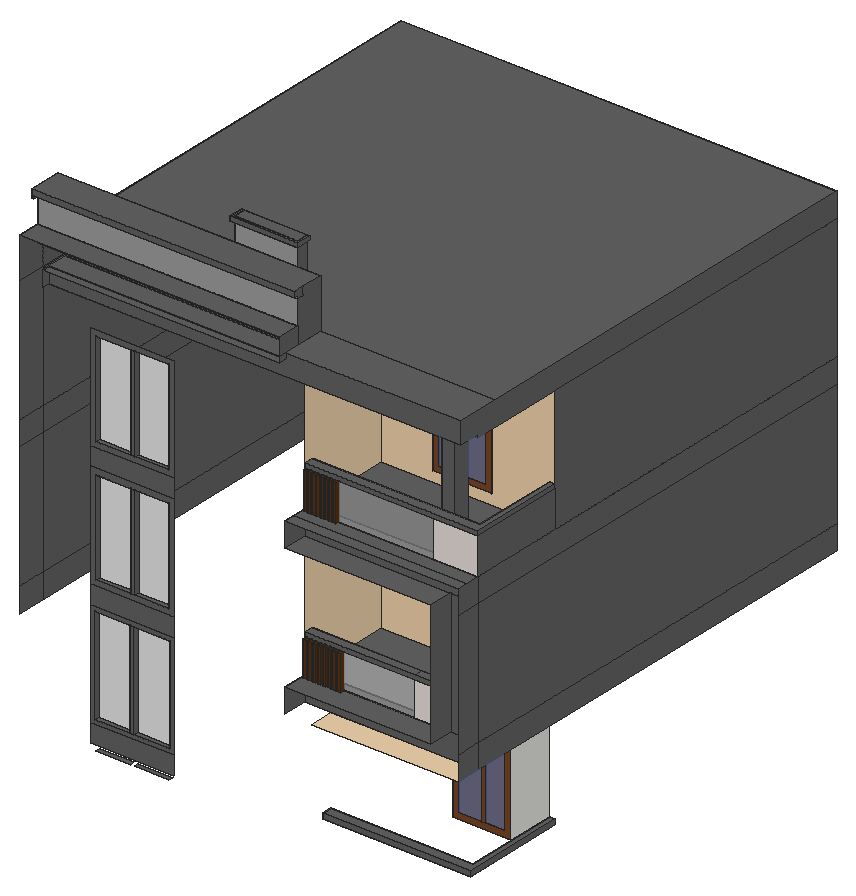
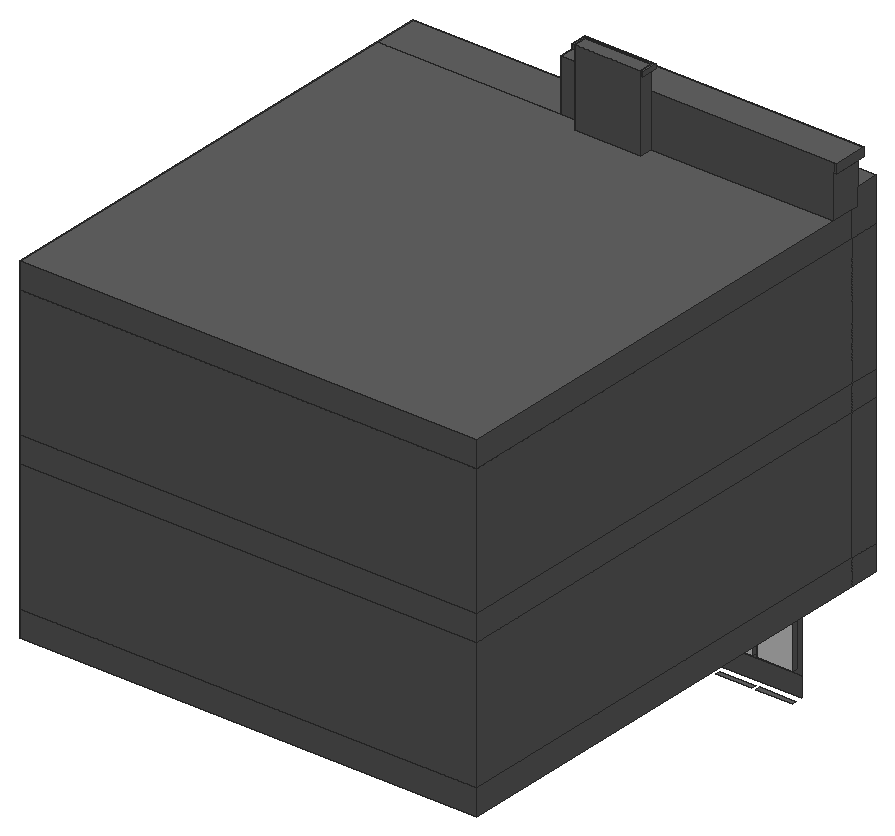
# SketchUp Ruby script. Lengths in inches.
U = 1.inch
M = Sketchup.active_model
def pt(a) = Geom::Point3d.new(a.map { |v| v * U })
def face(e, loops, mat)
  f = e.add_face(loops[0].map { |a| pt(a) })
  loops[1..].each { |l| e.add_face(l.map { |a| pt(a) }).erase! }
  f.material = f.back_material = mat if mat
  f
end
# faces: each face lists its corners as indices into pts; further lists are holes
def faces(e, pts, list, mat = nil) = list.each { |f| face(e, (f[0].is_a?(Array) ? f : [f]).map { |l| l.map { |i| pts[i] } }, mat) }
# xy, xz, yz: faces in a plane at the given z, y or x. An outline is a flat list of corners, or four numbers for a rectangle; further outlines are holes
def ring(l) = l.size == 4 ? [[l[0], l[1]], [l[2], l[1]], [l[2], l[3]], [l[0], l[3]]] : l.each_slice(2).to_a
def flat(e, list, mat, &to3) = list.each { |f| face(e, (f[0].is_a?(Array) ? f : [f]).map { |l| ring(l).map { |u, v| to3.(u, v) } }, mat) }
def xy(e, z, list, mat = nil) = flat(e, list, mat) { |x, y| [x, y, z] }
def xz(e, y, list, mat = nil) = flat(e, list, mat) { |x, z| [x, y, z] }
def yz(e, x, list, mat = nil) = flat(e, list, mat) { |y, z| [x, y, z] }
def lines(e, pts, list) = list.each { |a, b| e.add_line(pt(pts[a]), pt(pts[b])) }
# prism: a flat outline (further loops are holes) pulled along v
def prism(e, loops, v, mat = nil)
  f = face(e, loops, mat); d = Geom::Vector3d.new(v.map { |x| x * U })
  f.pushpull(f.normal.samedirection?(d) ? d.length : -d.length)
end
def box(e, o, s, mat = nil) = prism(e, [[o, [o[0] + s[0], o[1], o[2]], [o[0] + s[0], o[1] + s[1], o[2]], [o[0], o[1] + s[1], o[2]]]], [0, 0, s[2]], mat)
def at(x, y, z, deg = 0) = Geom::Transformation.translation(pt([x, y, z])) * Geom::Transformation.rotation(ORIGIN, Z_AXIS, deg.degrees)
def axes(o, x, y, z) = Geom::Transformation.new([*x, 0, *y, 0, *z, 0, *pt(o).to_a, 1])
def part(name) = M.definitions.add(name)
# library, detail: a bought-in or finely detailed component or shape, given as its bounding box
def library(name, o, s) = part(name).tap { |d| box(d.entities, o, s) }
def detail(e, o, s) = box(e.add_group.entities, o, s)
def put(e, d, t, mat = nil) = e.add_instance(d, t).tap { |i| i.material = mat if mat }
def group(e, t, mat = nil) = e.add_group.tap { |g| g.transformation = t; g.material = mat if mat }.entities
root = M.entities
M.materials.add("Generic\#1").color = [98, 98, 98]
M.materials.add("Generic\#2").color = [158, 158, 158]
M.materials.add("Generic\#3").color = [239, 209, 171]
M.materials.add("Generic\#4").color = [90, 50, 18]
M.materials.add("Generic\#5").color = [232, 223, 218]
M.materials.add("[Mirror 02]").color = [229, 229, 229]
M.materials.add("[Translucent Glass Blue]").color = [100, 149, 237]
M.materials["[Translucent Glass Blue]"].alpha = 0.5
M.materials.add("[Translucent Glass Gray]").color = [201, 201, 201]
M.materials["[Translucent Glass Gray]"].alpha = 0.5
M.materials.add("[Wood Veneer 01]").color = [120, 70, 37]
c1 = part("Group\#6")
xy(c1.entities,0,[[0,0,56.6875,3.1875]],"[Wood Veneer 01]")
xy(c1.entities,78.875,[[0,0,56.6875,3.1875]],"[Wood Veneer 01]")
xz(c1.entities,0,[[5.8,5.8,28.34,73.07],[31.82,5.8,50.88,73.07]],"[Translucent Glass Blue]")
xz(c1.entities,0,[[[0,0,56.6875,78.875],[5.8,5.8,50.88,73.07]],[28.34,5.8,31.82,73.07]],"[Wood Veneer 01]")
xz(c1.entities,3.1875,[[0,0,56.6875,78.875]],"[Wood Veneer 01]")
yz(c1.entities,0,[[0,0,3.1875,78.875]],"[Wood Veneer 01]")
yz(c1.entities,56.6875,[[0,0,3.1875,78.875]],"[Wood Veneer 01]")
c2 = part("Group\#2")
xy(c2.entities,33.25,[[0,0,3.3125,4.125]])
xz(c2.entities,0,[[0,0,3.3125,33.25]])
yz(c2.entities,0,[[0,0,4.125,33.25]])
yz(c2.entities,3.3125,[[0,0,4.125,33.25]])
c3 = part("Group\#3")
xy(c3.entities,35.375,[[0,0,3.1875,2.875]])
xz(c3.entities,0,[[0,0,3.1875,35.375]])
yz(c3.entities,0,[[0,0,2.875,35.375]])
yz(c3.entities,3.1875,[[0,0,2.875,35.375]])
xy(root,147.94,[[330.78,256.07,387.47,301.51]])
xy(root,150.73,[[61.12,163.51,94.41,167.88],[98.41,163.51,131.71,167.88]],"Generic\#1")
xy(root,176.0625,[[287.79,153.95,287.79,163.51,424.66,163.51,424.66,256.07,429.73,256.07,429.73,153.95]],"Generic\#1")
xy(root,177.67,[[60.27,163.51,93.5625,167.88],[97.5625,163.51,132.56,167.88]],"Generic\#1")
xy(root,180.875,[[287.79,153.95,429.73,153.95,429.73,256.07,424.66,256.07,424.66,163.51,287.79,163.51]],"Generic\#1")
xy(root,226.82,[[330.78,256.07,387.47,301.51]])
xy(root,263.5,[[287.79,139.95,429.73,163.51],[287.79,163.51,429.73,256.07]],"Generic\#3")
xy(root,271.21,[[60.27,163.51,93.5625,167.88],[97.5625,163.51,132.56,167.88]],"Generic\#1")
xy(root,287,[[262.1,139.95,403.16,139.95,403.16,163.51,267.48,163.51,267.48,159.38,264.16,159.38,264.16,163.51,262.1,163.51],[264.16,159.38,267.48,163.51],[262.1,163.51,403.16,172.01],[[262.1,172.01,403.16,256.07],[383.97,176.93,396.09,192.68]]],"Generic\#1")
xy(root,298.5,[[61.48,163.51,94.77,167.88],[98.77,163.51,131.35,167.88]],"Generic\#1")
xy(root,300.5,[[312.65,256.07,369.34,301.51]])
xy(root,320.25,[[262.1,163.51,403.16,172.01]],"Generic\#1")
xy(root,324.5,[[262.1,163.51,368.67,172.01],[368.67,163.51,403.16,172.01]],"Generic\#1")
xy(root,379.38,[[312.65,256.07,369.34,301.51]])
xy(root,389.62,[[61.48,163.51,94.77,167.88],[98.77,163.51,131.35,167.88]],"Generic\#1")
xy(root,407,[[262.1,139.95,403.16,163.51]],"Generic\#1")
xy(root,407,[[262.1,163.51,403.16,256.07]],"Generic\#3")
xy(root,417.99,[[61.34,163.51,94.63,167.88],[98.63,163.51,131.49,167.88]],"Generic\#1")
xy(root,430.5,[[262.1,139.95,429.73,150.2],[262.1,150.2,429.73,150.2,429.73,163.51,267.04,163.51,267.04,160.63,263.85,160.63,263.85,163.51,262.1,163.51],[263.85,160.63,267.04,163.51],[262.1,163.51,262.1,172.01,424.54,172.01,424.54,256.07,429.73,256.07,429.73,163.51],[262.1,172.01,424.54,256.07]],"Generic\#1")
xy(root,440.07,[[311.98,256.07,368.67,307.45]])
xy(root,465.875,[[262.1,163.51,262.1,172.01,424.54,172.01,424.54,256.07,429.73,256.07,429.73,163.51]],"Generic\#1")
xy(root,470.5,[[262.1,163.51,429.73,163.51,429.73,256.07,424.54,256.07,424.54,172.01,262.1,172.01]],"Generic\#1")
xy(root,509.39,[[61.34,163.51,94.63,167.88],[98.63,163.51,131.49,167.88]],"Generic\#1")
xy(root,518.94,[[311.98,256.07,368.67,307.45]])
xy(root,550.5,[[160.6,157.13,164.98,163.51],[166.98,157.13,171.35,163.51],[173.35,157.13,177.73,163.51],[179.73,157.13,184.1,163.51],[186.1,157.13,190.48,163.51],
  [192.48,157.13,196.85,163.51],[198.85,157.13,203.23,163.51],[205.23,157.13,209.6,163.51],[211.6,157.13,215.98,163.51],[217.98,157.13,222.35,163.51],
  [224.35,157.13,228.73,163.51],[230.73,157.13,235.1,163.51],[237.1,157.13,241.48,163.51],[243.48,157.13,247.85,163.51],[249.85,157.13,254.23,163.51],
  [256.23,157.13,260.6,163.51],[9.73,163.51,9.73,595.51,429.73,595.51,429.73,256.07,262.1,256.07,262.1,163.51]],"Generic\#1")
xy(root,550.5,[[262.1,163.51,429.73,256.07]],"Generic\#3")
xy(root,553.3125,[[32.23,143.07,262.1,163.51],[262.1,143.07,429.73,163.51]],"Generic\#1")
xy(root,568.125,[[32.23,136.13,260.65,143.07],[32.23,143.07,260.65,163.51],[260.65,143.07,262.1,163.51]],"Generic\#1")
xy(root,572.5,[[383.97,176.93,396.09,192.68]],"Generic\#1")
xy(root,574,[[260.65,143.07,429.73,184.76],[9.73,157.2,260.65,163.51],[9.73,163.51,260.65,184.76],[9.73,184.76,177.65,184.76,177.65,196.57,238.4,196.57,238.4,184.76,429.73,184.76,429.73,595.51,9.73,595.51],[177.65,184.76,238.4,196.57]],"Generic\#1")
xy(root,590.5625,[[9.73,136.13,260.65,157.2]],"Generic\#1")
xy(root,614,[[7.1,153.2,9.73,163.51],[9.73,157.2,260.65,163.51],[7.1,163.51,9.73,184.76]],"Generic\#1")
xy(root,616.5,[[9.73,153.2,260.65,157.2]],"Generic\#1")
xy(root,622.0625,[[7.1,153.2,260.65,184.76]],"Generic\#1")
xy(root,640.375,[[175.28,182.38,175.28,184.76,238.4,184.76,238.4,196.57,240.84,196.57,240.84,182.38],[175.28,184.76,177.65,196.57]],"Generic\#1")
xy(root,644.5,[[175.28,182.38,240.84,182.38,240.84,196.57,238.4,196.57,238.4,184.76,177.65,184.76,177.65,196.57,175.28,196.57],[177.65,184.76,238.4,196.57]],"Generic\#1")
xz(root,143.07,[[32.23,553.3125,429.73,553.3125,429.73,574,260.65,574,260.65,568.125,32.23,568.125]],"Generic\#1")
xz(root,153.2,[[7.1,614,9.73,614,9.73,616.5,260.65,616.5,260.65,622.0625,7.1,622.0625]],"Generic\#1")
xz(root,153.95,[[287.79,176.0625,429.73,180.875]],"Generic\#1")
xz(root,157.2,[[9.73,574,260.65,590.5625]],"Generic\#1")
xz(root,157.2,[[9.73,590.5625,260.65,614],[9.73,614,260.65,616.5]],"Generic\#2")
xz(root,163.51,[[56.23,155.625,136.6,173.625],[[56.23,173.625,136.6,275.25],[60.27,177.67,132.56,271.21]],[287.79,176.0625,395.15,180.875],[395.15,176.0625,424.66,180.875],[93.5625,177.67,97.5625,271.21],
  [262.1,263.5,429.73,287],[56.23,275.25,136.6,293.25],[262.1,287,264.16,320.25],[403.16,287,429.73,407],[[56.23,293.25,136.6,394.875],[61.48,298.5,131.35,389.62]],
  [94.77,298.5,98.77,389.62],[262.1,320.25,403.16,324.5],[56.23,394.875,136.6,412.875],[262.1,407,429.73,430.5],[[56.23,412.875,136.6,514.5],[61.34,417.99,131.49,509.39]],
  [94.63,417.99,98.63,509.39],[262.1,430.5,263.85,465.875],[262.1,465.875,429.73,470.5],[32.23,550.5,429.73,553.3125],[32.23,553.3125,262.1,568.125]],"Generic\#1")
xz(root,163.51,[[368.67,287,403.16,320.25],[386.74,430.5,429.73,465.875]],"Generic\#5")
xz(root,163.51,[[267.48,287,368.67,320.25],[267.04,430.5,386.74,465.875]],"[Translucent Glass Gray]")
xz(root,167.88,[[60.27,177.67,93.5625,271.21],[97.5625,177.67,132.56,271.21],[61.48,298.5,94.77,389.62],[98.77,298.5,131.35,389.62],[61.34,417.99,94.63,509.39],
  [98.63,417.99,131.49,509.39]],"[Mirror 02]")
xz(root,172.01,[[368.67,287,403.16,320.25],[262.1,320.25,368.67,324.5],[368.67,320.25,403.16,324.5],[262.1,430.5,386.74,465.875],[262.1,465.875,386.74,470.5],
  [386.74,465.875,424.54,470.5]],"Generic\#1")
xz(root,172.01,[[262.1,287,368.67,320.25],[386.74,430.5,424.54,465.875]],"[Translucent Glass Gray]")
xz(root,176.93,[[383.97,287,396.09,572.5]],"Generic\#1")
xz(root,182.38,[[175.28,640.375,240.84,644.5]],"Generic\#1")
xz(root,184.76,[[9.73,574,177.65,622.0625],[177.65,574,238.4,622.0625],[238.4,574,260.65,622.0625],[7.1,614,9.73,622.0625],[177.65,640.375,238.4,644.5]],"Generic\#1")
xz(root,184.76,[[177.65,622.0625,238.4,640.375]],"Generic\#2")
xz(root,192.68,[[383.97,287,396.09,572.5]],"Generic\#1")
xz(root,196.57,[[177.65,574,238.4,644.5],[175.28,640.375,177.65,644.5],[238.4,640.375,240.84,644.5]],"Generic\#1")
xz(root,256.07,[[[262.1,287,403.16,407],[312.65,300.5,369.34,379.38]],[[262.1,430.5,424.54,430.5,424.54,470.5,429.73,470.5,429.73,550.5,262.1,550.5],[311.98,440.07,368.67,518.94]]],"Generic\#3")
xz(root,301.51,[[330.78,147.94,387.47,226.82],[312.65,300.5,369.34,379.38]])
xz(root,307.45,[[311.98,440.07,368.67,518.94]])
xz(root,595.51,[[9.73,263.5,429.73,287],[9.73,287,429.73,407],[9.73,407,429.73,430.5],[9.73,430.5,429.73,550.5],[9.73,550.5,429.73,574]],"Generic\#1")
yz(root,7.1,[[153.2,614,184.76,622.0625]],"Generic\#1")
yz(root,9.73,[[136.13,263.5,163.51,287],[163.51,263.5,595.51,287],[136.13,287,163.51,407],[163.51,287,595.51,407],[136.13,407,163.51,430.5],
  [163.51,407,595.51,430.5],[136.13,430.5,163.51,550.5],[163.51,430.5,595.51,550.5],[136.13,550.5,136.13,590.5625,157.2,590.5625,157.2,574,163.51,574,163.51,550.5],[163.51,550.5,595.51,574],
  [157.2,574,184.76,614],[153.2,614,157.2,616.5]],"Generic\#1")
yz(root,32.23,[[136.13,553.3125,143.07,568.125]],"Generic\#1")
yz(root,60.27,[[163.51,177.67,167.88,271.21]],"Generic\#1")
yz(root,61.34,[[163.51,417.99,167.88,509.39]],"Generic\#1")
yz(root,61.48,[[163.51,298.5,167.88,389.62]],"Generic\#1")
yz(root,93.5625,[[163.51,177.67,167.88,271.21]],"Generic\#1")
yz(root,94.63,[[163.51,417.99,167.88,509.39]],"Generic\#1")
yz(root,94.77,[[163.51,298.5,167.88,389.62]],"Generic\#1")
yz(root,97.5625,[[163.51,177.67,167.88,271.21]],"Generic\#1")
yz(root,98.63,[[163.51,417.99,167.88,509.39]],"Generic\#1")
yz(root,98.77,[[163.51,298.5,167.88,389.62]],"Generic\#1")
yz(root,131.35,[[163.51,298.5,167.88,389.62]],"Generic\#1")
yz(root,131.49,[[163.51,417.99,167.88,509.39]],"Generic\#1")
yz(root,132.56,[[163.51,177.67,167.88,271.21]],"Generic\#1")
yz(root,175.28,[[182.38,640.375,196.57,644.5]],"Generic\#1")
yz(root,177.65,[[184.76,574,196.57,640.375],[184.76,640.375,196.57,644.5]],"Generic\#1")
yz(root,238.4,[[184.76,574,196.57,640.375],[184.76,640.375,196.57,644.5]],"Generic\#1")
yz(root,240.84,[[182.38,640.375,196.57,644.5]],"Generic\#1")
yz(root,260.65,[[136.13,568.125,143.07,574],[136.13,574,157.2,590.5625],[157.2,574,184.76,574,184.76,622.0625,163.51,622.0625,163.51,614,157.2,614],[157.2,614,163.51,614,163.51,622.0625,153.2,622.0625,153.2,616.5,157.2,616.5]],"Generic\#1")
yz(root,262.1,[[139.95,263.5,163.51,287],[163.51,287,172.01,320.25],[163.51,320.25,172.01,324.5],[139.95,407,163.51,430.5],[163.51,430.5,172.01,465.875],
  [163.51,465.875,172.01,470.5]],"Generic\#1")
yz(root,262.1,[[172.01,287,256.07,287,256.07,407,163.51,407,163.51,324.5,172.01,324.5],[172.01,430.5,256.07,430.5,256.07,550.5,163.51,550.5,163.51,470.5,172.01,470.5]],"Generic\#3")
yz(root,287.79,[[153.95,176.0625,163.51,180.875]],"Generic\#1")
yz(root,311.98,[[256.07,440.07,307.45,518.94]])
yz(root,312.65,[[256.07,300.5,301.51,379.38]])
yz(root,330.78,[[256.07,147.94,301.51,226.82]])
yz(root,368.67,[[256.07,440.07,307.45,518.94]])
yz(root,369.34,[[256.07,300.5,301.51,379.38]])
yz(root,383.97,[[176.93,287,192.68,572.5]],"Generic\#1")
yz(root,387.47,[[256.07,147.94,301.51,226.82]])
yz(root,396.09,[[176.93,287,192.68,572.5]],"Generic\#1")
yz(root,403.16,[[139.95,287,163.51,407],[163.51,287,172.01,320.25],[172.01,287,172.01,324.5,163.51,324.5,163.51,407,256.07,407,256.07,287],[163.51,320.25,172.01,324.5]],"Generic\#1")
yz(root,424.54,[[172.01,430.5,256.07,465.875],[172.01,465.875,256.07,470.5]],"Generic\#1")
yz(root,424.66,[[163.51,176.0625,256.07,180.875]],"Generic\#1")
yz(root,429.73,[[153.95,176.0625,256.07,180.875],[139.95,263.5,163.51,287],[163.51,263.5,595.51,287],[139.95,287,163.51,407],[163.51,287,595.51,407],
  [139.95,407,163.51,430.5],[163.51,407,595.51,430.5],[163.51,430.5,256.07,465.875],[256.07,430.5,595.51,550.5],[163.51,465.875,256.07,470.5],
  [163.51,550.5,595.51,550.5,595.51,574,143.07,574,143.07,553.3125,163.51,553.3125]],"Generic\#1")
p = [[9.73,163.51,614],[9.73,163.51,616.9375]]
lines(root,p,[[0,1]])
put(root,c1,at(330.78,256.07,147.94))
put(root,c2,at(264.16,159.38,287),"Generic\#4")
put(root,c2,at(268.85,159.38,287),"Generic\#4")
put(root,c2,at(273.54,159.38,287),"Generic\#4")
put(root,c2,at(278.23,159.38,287),"Generic\#4")
put(root,c2,at(282.91,159.38,287),"Generic\#4")
put(root,c2,at(287.6,159.38,287),"Generic\#4")
put(root,c2,at(292.29,159.38,287),"Generic\#4")
put(root,c2,at(296.98,159.38,287),"Generic\#4")
put(root,c1,at(312.65,256.07,300.5))
put(root,c3,at(263.85,160.63,430.5),"Generic\#4")
put(root,c3,at(267.85,160.63,430.5),"Generic\#4")
put(root,c3,at(271.85,160.63,430.5),"Generic\#4")
put(root,c3,at(275.85,160.63,430.5),"Generic\#4")
put(root,c3,at(279.85,160.63,430.5),"Generic\#4")
put(root,c3,at(283.85,160.63,430.5),"Generic\#4")
put(root,c3,at(287.85,160.63,430.5),"Generic\#4")
put(root,c3,at(291.85,160.63,430.5),"Generic\#4")
put(root,c1,at(311.98,256.07,440.07))
